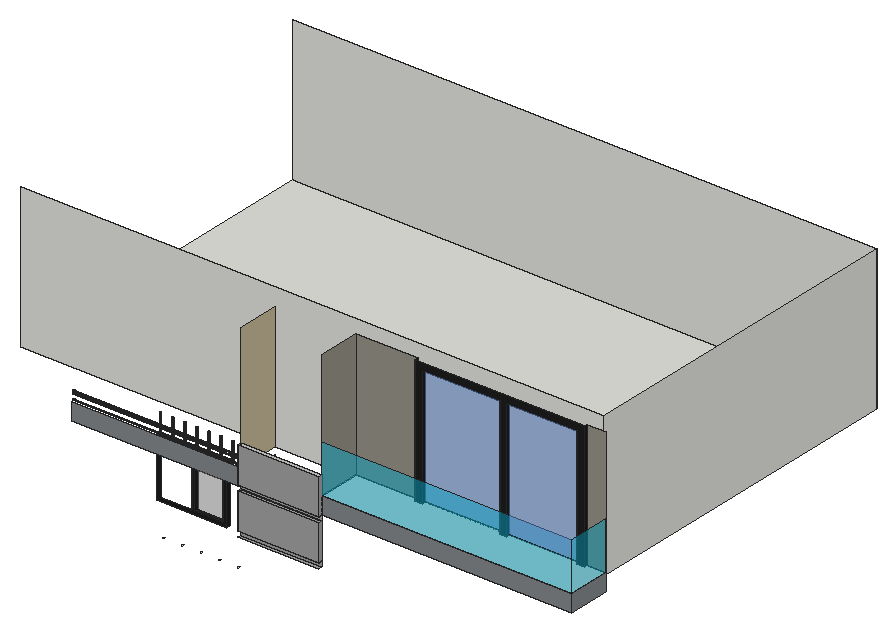
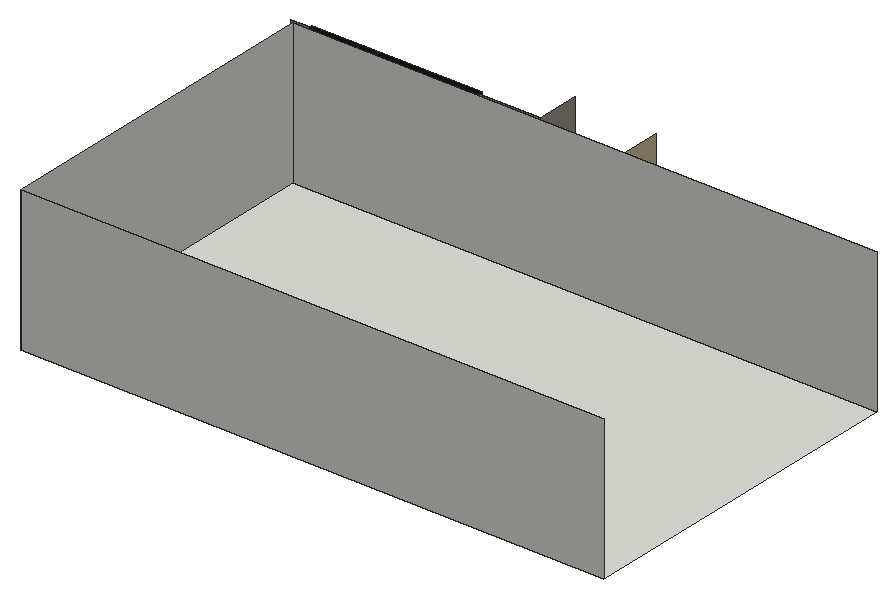
# SketchUp Ruby script. Lengths in inches.
U = 1.inch
M = Sketchup.active_model
def pt(a) = Geom::Point3d.new(a.map { |v| v * U })
def face(e, loops, mat)
  f = e.add_face(loops[0].map { |a| pt(a) })
  loops[1..].each { |l| e.add_face(l.map { |a| pt(a) }).erase! }
  f.material = f.back_material = mat if mat
  f
end
# faces: each face lists its corners as indices into pts; further lists are holes
def faces(e, pts, list, mat = nil) = list.each { |f| face(e, (f[0].is_a?(Array) ? f : [f]).map { |l| l.map { |i| pts[i] } }, mat) }
# xy, xz, yz: faces in a plane at the given z, y or x. An outline is a flat list of corners, or four numbers for a rectangle; further outlines are holes
def ring(l) = l.size == 4 ? [[l[0], l[1]], [l[2], l[1]], [l[2], l[3]], [l[0], l[3]]] : l.each_slice(2).to_a
def flat(e, list, mat, &to3) = list.each { |f| face(e, (f[0].is_a?(Array) ? f : [f]).map { |l| ring(l).map { |u, v| to3.(u, v) } }, mat) }
def xy(e, z, list, mat = nil) = flat(e, list, mat) { |x, y| [x, y, z] }
def xz(e, y, list, mat = nil) = flat(e, list, mat) { |x, z| [x, y, z] }
def yz(e, x, list, mat = nil) = flat(e, list, mat) { |y, z| [x, y, z] }
def lines(e, pts, list) = list.each { |a, b| e.add_line(pt(pts[a]), pt(pts[b])) }
# prism: a flat outline (further loops are holes) pulled along v
def prism(e, loops, v, mat = nil)
  f = face(e, loops, mat); d = Geom::Vector3d.new(v.map { |x| x * U })
  f.pushpull(f.normal.samedirection?(d) ? d.length : -d.length)
end
def box(e, o, s, mat = nil) = prism(e, [[o, [o[0] + s[0], o[1], o[2]], [o[0] + s[0], o[1] + s[1], o[2]], [o[0], o[1] + s[1], o[2]]]], [0, 0, s[2]], mat)
def at(x, y, z, deg = 0) = Geom::Transformation.translation(pt([x, y, z])) * Geom::Transformation.rotation(ORIGIN, Z_AXIS, deg.degrees)
def axes(o, x, y, z) = Geom::Transformation.new([*x, 0, *y, 0, *z, 0, *pt(o).to_a, 1])
def part(name) = M.definitions.add(name)
# library, detail: a bought-in or finely detailed component or shape, given as its bounding box
def library(name, o, s) = part(name).tap { |d| box(d.entities, o, s) }
def detail(e, o, s) = box(e.add_group.entities, o, s)
def put(e, d, t, mat = nil) = e.add_instance(d, t).tap { |i| i.material = mat if mat }
def group(e, t, mat = nil) = e.add_group.tap { |g| g.transformation = t; g.material = mat if mat }.entities
root = M.entities
M.materials.add("[0133_Gray]").color = [128, 128, 128]
M.materials.add("[Blacktop New]").color = [30, 30, 30]
M.materials.add("[Blacktop Old 01]").color = [132, 136, 139]
M.materials.add("[Formica Graystone]").color = [149, 146, 135]
M.materials.add("[Marble Carrara Gold Floor Tile]").color = [225, 223, 217]
M.materials.add("[Pavers Flagstone Gray]").color = [162, 162, 162]
M.materials.add("[Quartz Light Brown]").color = [199, 184, 152]
M.materials.add("[Translucent Glass Blue]").color = [100, 149, 237]
M.materials["[Translucent Glass Blue]"].alpha = 0.5
M.materials.add("[Translucent Glass Gray]").color = [128, 128, 128]
M.materials["[Translucent Glass Gray]"].alpha = 0.5
M.materials.add("[Translucent Glass Tinted]").color = [8, 201, 241]
M.materials["[Translucent Glass Tinted]"].alpha = 0.48
xy(root,170.77,[[164.56,3.4,164.7,3.4,164.82,3.44,164.93,3.52,165.01,3.61,165.07,3.73,165.1,3.86,165.09,3.99,165.05,4.11,164.98,4.22,164.88,4.31,164.76,4.37,164.64,4.39,164.51,4.39,164.38,4.34,164.27,4.27,164.1875,4.18,164.13,4.06,164.1,3.93,164.11,3.8,164.15,3.68,164.22,3.57,164.32,3.48,164.4375,3.42],[180.19,3.4,180.32,3.4,180.44,3.44,180.55,3.52,180.64,3.61,180.7,3.73,180.72,3.86,180.72,3.99,180.68,4.11,180.6,4.22,180.51,4.31,180.39,4.37,180.26,4.39,180.13,4.39,180.01,4.34,179.9,4.27,179.8125,4.18,179.75,4.06,179.73,3.93,179.73,3.8,179.78,3.68,179.85,3.57,179.95,3.48,180.0625,3.42],[195.81,3.4,195.95,3.4,196.07,3.44,196.18,3.52,196.26,3.61,196.32,3.73,196.35,3.86,196.34,3.99,196.3,4.11,196.23,4.22,196.13,4.31,196.01,4.37,195.89,4.39,195.76,4.39,195.63,4.34,195.52,4.27,195.4375,4.18,195.38,4.06,195.35,3.93,195.36,3.8,195.4,3.68,195.47,3.57,195.57,3.48,195.6875,3.42],[211.44,3.4,211.57,3.4,211.69,3.44,211.8,3.52,211.89,3.61,211.95,3.73,211.97,3.86,211.97,3.99,211.93,4.11,211.85,4.22,211.76,4.31,211.64,4.37,211.51,4.39,211.38,4.39,211.26,4.34,211.15,4.27,211.0625,4.18,211,4.06,210.98,3.93,210.98,3.8,211.03,3.68,211.1,3.57,211.2,3.48,211.3125,3.42],[227.06,3.4,227.2,3.4,227.32,3.44,227.43,3.52,227.51,3.61,227.57,3.73,227.6,3.86,227.59,3.99,227.55,4.11,227.48,4.22,227.38,4.31,227.26,4.37,227.14,4.39,227.01,4.39,226.88,4.34,226.77,4.27,226.6875,4.18,226.63,4.06,226.6,3.93,226.61,3.8,226.65,3.68,226.72,3.57,226.82,3.48,226.9375,3.42]])
xy(root,173.78,[[133.06,36,191.5,39]],"[Blacktop New]")
xy(root,176.78,[[164.73,36,188.5,39]],"[Blacktop New]")
xy(root,195.875,[[229.62,0,297.58,3]],"[Pavers Flagstone Gray]")
xy(root,200.56,[[229.62,0,297.58,3]],"[Pavers Flagstone Gray]")
xy(root,220.84,[[164.73,36,188.5,39]],"[Blacktop New]")
xy(root,223.84,[[133.06,36,191.5,39]],"[Blacktop New]")
xy(root,229.1875,[[420.16,36,423.8,39]])
xy(root,229.1875,[[355.33,36,420.16,39],[423.8,36,485,39]],"[Blacktop New]")
xy(root,230.4375,[[229.62,0,297.58,3]],"[Pavers Flagstone Gray]")
xy(root,235.12,[[229.62,0,297.58,3]],"[Pavers Flagstone Gray]")
xy(root,235.1875,[[349.33,36,491,39]])
xy(root,235.1875,[[297.58,3,297.58,39,349.33,39,349.33,36,491,36,491,39,506.625,39,506.625,3]],"[Blacktop Old 01]")
xy(root,240,[[9,48,497.625,333.4375]])
xy(root,246.23,[[231.98,3.83,232.14,3.85,232.29,3.92,232.42,4.02,232.52,4.15,232.58,4.3,232.6,4.46,232.58,4.62,232.52,4.77,232.42,4.9,232.29,5,232.14,5.0625,231.98,5.08,231.82,5.0625,231.67,5,231.54,4.9,231.4375,4.77,231.375,4.62,231.35,4.46,231.375,4.3,231.4375,4.15,231.54,4.02,231.67,3.92,231.82,3.85],[242.1,3.83,242.27,3.85,242.42,3.92,242.55,4.02,242.65,4.15,242.71,4.3,242.73,4.46,242.71,4.62,242.65,4.77,242.55,4.9,242.42,5,242.27,5.0625,242.1,5.08,241.94,5.0625,241.79,5,241.66,4.9,241.5625,4.77,241.5,4.62,241.48,4.46,241.5,4.3,241.5625,4.15,241.66,4.02,241.79,3.92,241.94,3.85],[252.23,3.83,252.39,3.85,252.54,3.92,252.67,4.02,252.77,4.15,252.83,4.3,252.85,4.46,252.83,4.62,252.77,4.77,252.67,4.9,252.54,5,252.39,5.0625,252.23,5.08,252.07,5.0625,251.92,5,251.79,4.9,251.6875,4.77,251.625,4.62,251.6,4.46,251.625,4.3,251.6875,4.15,251.79,4.02,251.92,3.92,252.07,3.85],[262.35,3.83,262.52,3.85,262.67,3.92,262.8,4.02,262.9,4.15,262.96,4.3,262.98,4.46,262.96,4.62,262.9,4.77,262.8,4.9,262.67,5,262.52,5.0625,262.35,5.08,262.19,5.0625,262.04,5,261.91,4.9,261.8125,4.77,261.75,4.62,261.73,4.46,261.75,4.3,261.8125,4.15,261.91,4.02,262.04,3.92,262.19,3.85]])
xy(root,249.45,[[349.33,36,355.33,39],[420.16,36,425.68,39],[485,36,491,39]])
xy(root,249.45,[[297.58,3,506.625,3,506.625,39,491,39,491,36,485,36,485,39,425.68,39,425.68,36,420.16,36,420.16,39,355.33,39,355.33,36,349.33,36,349.33,39,297.58,39]],"[Marble Carrara Gold Floor Tile]")
xz(root,0,[[229.62,200.56,297.58,230.4375],[229.62,235.12,297.58,265]],"[Pavers Flagstone Gray]")
xz(root,3,[[229.62,200.56,297.58,230.4375],[229.62,235.12,297.58,265]])
xz(root,3,[[88.53,232,229.62,246.23],[297.58,235.1875,506.625,249.45]],"[Blacktop Old 01]")
xz(root,3,[[229.62,195.875,297.58,200.56],[229.62,230.4375,297.58,235.12]],"[Pavers Flagstone Gray]")
xz(root,3,[[297.58,249.45,506.625,290.01]],"[Translucent Glass Tinted]")
xz(root,36,[[[133.06,173.78,191.5,223.84],[136.06,176.78,162.28,220.84],[164.73,176.78,188.5,220.84]],[349.33,249.45,355.33,249.45,355.33,349.1875,420.16,349.1875,420.16,249.45,425.68,249.45,425.68,349.1875,485,349.1875,485,249.45,491,249.45,491,355.1875,349.33,355.1875]],"[Blacktop New]")
xz(root,39,[[297.58,235.1875,506.625,239.9375],[297.58,239.9375,506.625,249.45]])
xz(root,39,[[297.58,249.45,349.33,355.1875],[491,249.45,506.625,355.1875]],"[Formica Graystone]")
xz(root,39,[[355.33,249.45,420.16,349.1875],[425.68,249.45,485,349.1875]],"[Translucent Glass Blue]")
xz(root,39,[[164.73,176.78,188.5,220.84]],"[Translucent Glass Gray]")
xz(root,48,[[9,240,497.625,360]])
xz(root,333.4375,[[9,240,497.625,360]])
yz(root,162.28,[[36,176.78,39,220.84]],"[Blacktop New]")
yz(root,164.73,[[36,176.78,39,220.84]],"[Blacktop New]")
yz(root,188.5,[[36,176.78,39,220.84]],"[Blacktop New]")
yz(root,191.5,[[36,173.78,39,223.84]],"[Blacktop New]")
yz(root,229.62,[[3,232,39,240],[3,240,39,240.1875]])
yz(root,229.62,[[0,200.56,3,230.4375],[0,235.12,3,265]],"[Pavers Flagstone Gray]")
yz(root,229.62,[[[3,246.23,39,351.5625],[3.53,262.01,3.625,262.03,3.71,262.0625,3.79,262.12,3.85,262.2,3.89,262.29,3.9,262.39,3.89,262.48,3.85,262.58,3.79,262.65,3.71,262.71,3.625,262.75,3.53,262.76,3.43,262.75,3.34,262.71,3.26,262.65,3.2,262.58,3.16,262.48,3.15,262.39,3.16,262.29,3.2,262.2,3.26,262.12,3.34,262.0625,3.43,262.03],[3.53,260.45,3.625,260.46,3.71,260.5,3.79,260.56,3.85,260.64,3.89,260.73,3.9,260.83,3.89,260.92,3.85,261.01,3.79,261.09,3.71,261.15,3.625,261.1875,3.53,261.2,3.43,261.1875,3.34,261.15,3.26,261.09,3.2,261.01,3.16,260.92,3.15,260.83,3.16,260.73,3.2,260.64,3.26,260.56,3.34,260.5,3.43,260.46],[3.53,258.89,3.625,258.9,3.71,258.9375,3.79,259,3.85,259.08,3.89,259.17,3.9,259.26,3.89,259.36,3.85,259.45,3.79,259.53,3.71,259.59,3.625,259.625,3.53,259.64,3.43,259.625,3.34,259.59,3.26,259.53,3.2,259.45,3.16,259.36,3.15,259.26,3.16,259.17,3.2,259.08,3.26,259,3.34,258.9375,3.43,258.9],[3.53,257.33,3.625,257.34,3.71,257.375,3.79,257.43,3.85,257.51,3.89,257.6,3.9,257.7,3.89,257.8,3.85,257.89,3.79,257.97,3.71,258.02,3.625,258.0625,3.53,258.08,3.43,258.0625,3.34,258.02,3.26,257.97,3.2,257.89,3.16,257.8,3.15,257.7,3.16,257.6,3.2,257.51,3.26,257.43,3.34,257.375,3.43,257.34],[3.53,249.51,3.625,249.53,3.71,249.5625,3.79,249.62,3.85,249.7,3.89,249.79,3.9,249.89,3.89,249.98,3.85,250.08,3.79,250.15,3.71,250.21,3.625,250.25,3.53,250.26,3.43,250.25,3.34,250.21,3.26,250.15,3.2,250.08,3.16,249.98,3.15,249.89,3.16,249.79,3.2,249.7,3.26,249.62,3.34,249.5625,3.43,249.53],[3.53,251.08,3.625,251.09,3.71,251.125,3.79,251.18,3.85,251.26,3.89,251.35,3.9,251.45,3.89,251.55,3.85,251.64,3.79,251.72,3.71,251.77,3.625,251.8125,3.53,251.83,3.43,251.8125,3.34,251.77,3.26,251.72,3.2,251.64,3.16,251.55,3.15,251.45,3.16,251.35,3.2,251.26,3.26,251.18,3.34,251.125,3.43,251.09]]],"[Quartz Light Brown]")
yz(root,229.85,[[3.53,255.76,3.625,255.78,3.71,255.8125,3.79,255.87,3.85,255.95,3.89,256.04,3.9,256.14,3.89,256.23,3.85,256.33,3.79,256.4,3.71,256.46,3.625,256.5,3.53,256.51,3.43,256.5,3.34,256.46,3.26,256.4,3.2,256.33,3.16,256.23,3.15,256.14,3.16,256.04,3.2,255.95,3.26,255.87,3.34,255.8125,3.43,255.78]])
yz(root,231.78,[[3.53,254.2,3.625,254.21,3.71,254.25,3.79,254.31,3.85,254.39,3.89,254.48,3.9,254.58,3.89,254.67,3.85,254.76,3.79,254.84,3.71,254.9,3.625,254.9375,3.53,254.95,3.43,254.9375,3.34,254.9,3.26,254.84,3.2,254.76,3.16,254.67,3.15,254.58,3.16,254.48,3.2,254.39,3.26,254.31,3.34,254.25,3.43,254.21]])
yz(root,231.85,[[3.53,252.64,3.625,252.65,3.71,252.6875,3.79,252.75,3.85,252.83,3.89,252.92,3.9,253.01,3.89,253.11,3.85,253.2,3.79,253.28,3.71,253.34,3.625,253.375,3.53,253.39,3.43,253.375,3.34,253.34,3.26,253.28,3.2,253.2,3.16,253.11,3.15,253.01,3.16,252.92,3.2,252.83,3.26,252.75,3.34,252.6875,3.43,252.65]])
yz(root,232.16,[[3.53,247.95,3.625,247.96,3.71,248,3.79,248.06,3.85,248.14,3.89,248.23,3.9,248.33,3.89,248.42,3.85,248.51,3.79,248.59,3.71,248.65,3.625,248.6875,3.53,248.7,3.43,248.6875,3.34,248.65,3.26,248.59,3.2,248.51,3.16,248.42,3.15,248.33,3.16,248.23,3.2,248.14,3.26,248.06,3.34,248,3.43,247.96]])
yz(root,297.58,[[0,200.56,3,200.625],[0,235.12,3,235.1875],[3,235.1875,39,249.45]])
yz(root,297.58,[[3,249.45,39,355.1875]],"[Formica Graystone]")
yz(root,297.58,[[0,200.625,3,230.4375],[0,235.1875,3,265]],"[Pavers Flagstone Gray]")
yz(root,349.33,[[36,249.45,39,355.1875]],"[Blacktop New]")
yz(root,355.33,[[36,249.45,39,349.1875]],"[Blacktop New]")
yz(root,420.16,[[36,249.45,39,349.1875]],"[Blacktop New]")
yz(root,425.68,[[36,249.45,39,349.1875]],"[Blacktop New]")
yz(root,485,[[36,249.45,39,349.1875]],"[Blacktop New]")
yz(root,491,[[36,249.45,39,355.1875]],"[Blacktop New]")
yz(root,497.625,[[48,240,333.4375,360]])
yz(root,506.625,[[3,235.1875,39,249.45]],"[Blacktop Old 01]")
yz(root,506.625,[[3,249.45,39,290.04]],"[Translucent Glass Tinted]")
p = [[160.94,3.85,246.23],[161.1,3.83,246.23],[161.1,3.83,263.16],[160.94,3.85,263.16],[161.27,3.85,246.23],[161.27,3.85,263.16],
  [171.07,3.85,246.23],[171.23,3.83,246.23],[171.23,3.83,263.16],[171.07,3.85,263.16],[171.39,3.85,246.23],[171.39,3.85,263.16],
  [181.19,3.85,246.23],[181.35,3.83,246.23],[181.35,3.83,263.16],[181.19,3.85,263.16],[181.52,3.85,246.23],[181.52,3.85,263.16],
  [191.32,3.85,246.23],[191.48,3.83,246.23],[191.48,3.83,263.16],[191.32,3.85,263.16],[191.64,3.85,246.23],[191.64,3.85,263.16],
  [201.44,3.85,246.23],[201.6,3.83,246.23],[201.6,3.83,263.16],[201.44,3.85,263.16],[201.77,3.85,246.23],[201.77,3.85,263.16],
  [211.57,3.85,246.23],[211.73,3.83,246.23],[211.73,3.83,263.16],[211.57,3.85,263.16],[211.89,3.85,246.23],[211.89,3.85,263.16],
  [221.69,3.85,246.23],[221.85,3.83,246.23],[221.85,3.83,263.16],[221.69,3.85,263.16],[222.02,3.85,246.23],[222.02,3.85,263.16],
  [160.66,4.02,246.23],[160.79,3.92,246.23],[160.79,3.92,263.16],[160.66,4.02,263.16],[161.42,3.92,246.23],[161.42,3.92,263.16],
  [161.55,4.02,246.23],[161.55,4.02,263.16],[170.79,4.02,246.23],[170.92,3.92,246.23],[170.92,3.92,263.16],[170.79,4.02,263.16],
  [171.54,3.92,246.23],[171.54,3.92,263.16],[171.67,4.02,246.23],[171.67,4.02,263.16],[180.91,4.02,246.23],[181.04,3.92,246.23],
  [181.04,3.92,263.16],[180.91,4.02,263.16],[181.67,3.92,246.23],[181.67,3.92,263.16],[181.8,4.02,246.23],[181.8,4.02,263.16],
  [191.04,4.02,246.23],[191.17,3.92,246.23],[191.17,3.92,263.16],[191.04,4.02,263.16],[191.79,3.92,246.23],[191.79,3.92,263.16],
  [191.92,4.02,246.23],[191.92,4.02,263.16],[201.16,4.02,246.23],[201.29,3.92,246.23],[201.29,3.92,263.16],[201.16,4.02,263.16],
  [201.92,3.92,246.23],[201.92,3.92,263.16],[202.05,4.02,246.23],[202.05,4.02,263.16],[211.29,4.02,246.23],[211.42,3.92,246.23],
  [211.42,3.92,263.16],[211.29,4.02,263.16],[212.04,3.92,246.23],[212.04,3.92,263.16],[212.17,4.02,246.23],[212.17,4.02,263.16],
  [221.41,4.02,246.23],[221.54,3.92,246.23],[221.54,3.92,263.16],[221.41,4.02,263.16],[222.17,3.92,246.23],[222.17,3.92,263.16],
  [222.3,4.02,246.23],[222.3,4.02,263.16],[160.5625,4.15,246.23],[160.5625,4.15,263.16],[161.65,4.15,246.23],[161.65,4.15,263.16],
  [170.6875,4.15,246.23],[170.6875,4.15,263.16],[171.77,4.15,246.23],[171.77,4.15,263.16],[180.8125,4.15,246.23],[180.8125,4.15,263.16],
  [181.9,4.15,246.23],[181.9,4.15,263.16],[190.9375,4.15,246.23],[190.9375,4.15,263.16],[192.02,4.15,246.23],[192.02,4.15,263.16],
  [201.0625,4.15,246.23],[201.0625,4.15,263.16],[202.15,4.15,246.23],[202.15,4.15,263.16],[211.1875,4.15,246.23],[211.1875,4.15,263.16],
  [212.27,4.15,246.23],[212.27,4.15,263.16],[221.3125,4.15,246.23],[221.3125,4.15,263.16],[222.4,4.15,246.23],[222.4,4.15,263.16],
  [160.5,4.3,246.23],[160.5,4.3,263.16],[161.71,4.3,246.23],[161.71,4.3,263.16],[170.625,4.3,246.23],[170.625,4.3,263.16],
  [171.83,4.3,246.23],[171.83,4.3,263.16],[180.75,4.3,246.23],[180.75,4.3,263.16],[181.96,4.3,246.23],[181.96,4.3,263.16],
  [190.875,4.3,246.23],[190.875,4.3,263.16],[192.08,4.3,246.23],[192.08,4.3,263.16],[201,4.3,246.23],[201,4.3,263.16],
  [202.21,4.3,246.23],[202.21,4.3,263.16],[211.125,4.3,246.23],[211.125,4.3,263.16],[212.33,4.3,246.23],[212.33,4.3,263.16],
  [221.25,4.3,246.23],[221.25,4.3,263.16],[222.46,4.3,246.23],[222.46,4.3,263.16],[160.48,4.46,246.23],[160.48,4.46,263.16],
  [161.73,4.46,246.23],[161.73,4.46,263.16],[170.6,4.46,246.23],[170.6,4.46,263.16],[171.85,4.46,246.23],[171.85,4.46,263.16],
  [180.73,4.46,246.23],[180.73,4.46,263.16],[181.98,4.46,246.23],[181.98,4.46,263.16],[190.85,4.46,246.23],[190.85,4.46,263.16],
  [192.1,4.46,246.23],[192.1,4.46,263.16],[200.98,4.46,246.23],[200.98,4.46,263.16],[202.23,4.46,246.23],[202.23,4.46,263.16],
  [211.1,4.46,246.23],[211.1,4.46,263.16],[212.35,4.46,246.23],[212.35,4.46,263.16],[221.23,4.46,246.23],[221.23,4.46,263.16],
  [222.48,4.46,246.23],[222.48,4.46,263.16],[160.5,4.62,246.23],[160.5,4.62,263.16],[161.71,4.62,246.23],[161.71,4.62,263.16],
  [170.625,4.62,246.23],[170.625,4.62,263.16],[171.83,4.62,246.23],[171.83,4.62,263.16],[180.75,4.62,246.23],[180.75,4.62,263.16],
  [181.96,4.62,246.23],[181.96,4.62,263.16],[190.875,4.62,246.23],[190.875,4.62,263.16],[192.08,4.62,246.23],[192.08,4.62,263.16],
  [201,4.62,246.23],[201,4.62,263.16],[202.21,4.62,246.23],[202.21,4.62,263.16],[211.125,4.62,246.23],[211.125,4.62,263.16],
  [212.33,4.62,246.23],[212.33,4.62,263.16],[221.25,4.62,246.23],[221.25,4.62,263.16],[222.46,4.62,246.23],[222.46,4.62,263.16],
  [160.5625,4.77,246.23],[160.5625,4.77,263.16],[161.65,4.77,246.23],[161.65,4.77,263.16],[170.6875,4.77,246.23],[170.6875,4.77,263.16],
  [171.77,4.77,246.23],[171.77,4.77,263.16],[180.8125,4.77,246.23],[180.8125,4.77,263.16],[181.9,4.77,246.23],[181.9,4.77,263.16],
  [190.9375,4.77,246.23],[190.9375,4.77,263.16],[192.02,4.77,246.23],[192.02,4.77,263.16],[201.0625,4.77,246.23],[201.0625,4.77,263.16],
  [202.15,4.77,246.23],[202.15,4.77,263.16],[211.1875,4.77,246.23],[211.1875,4.77,263.16],[212.27,4.77,246.23],[212.27,4.77,263.16],
  [221.3125,4.77,246.23],[221.3125,4.77,263.16],[222.4,4.77,246.23],[222.4,4.77,263.16],[160.66,4.9,246.23],[160.66,4.9,263.16],
  [161.55,4.9,246.23],[161.55,4.9,263.16],[170.79,4.9,246.23],[170.79,4.9,263.16],[171.67,4.9,246.23],[171.67,4.9,263.16],
  [180.91,4.9,246.23],[180.91,4.9,263.16],[181.8,4.9,246.23],[181.8,4.9,263.16],[191.04,4.9,246.23],[191.04,4.9,263.16],
  [191.92,4.9,246.23],[191.92,4.9,263.16],[201.16,4.9,246.23],[201.16,4.9,263.16],[202.05,4.9,246.23],[202.05,4.9,263.16],
  [211.29,4.9,246.23],[211.29,4.9,263.16],[212.17,4.9,246.23],[212.17,4.9,263.16],[221.41,4.9,246.23],[221.41,4.9,263.16],
  [222.3,4.9,246.23],[222.3,4.9,263.16],[160.79,5,246.23],[160.79,5,263.16],[161.42,5,246.23],[161.42,5,263.16],
  [170.92,5,246.23],[170.92,5,263.16],[171.54,5,246.23],[171.54,5,263.16],[181.04,5,246.23],[181.04,5,263.16],
  [181.67,5,246.23],[181.67,5,263.16],[191.17,5,246.23],[191.17,5,263.16],[191.79,5,246.23],[191.79,5,263.16],
  [201.29,5,246.23],[201.29,5,263.16],[201.92,5,246.23],[201.92,5,263.16],[211.42,5,246.23],[211.42,5,263.16],
  [212.04,5,246.23],[212.04,5,263.16],[221.54,5,246.23],[221.54,5,263.16],[222.17,5,246.23],[222.17,5,263.16],
  [160.94,5.0625,246.23],[160.94,5.0625,263.16],[161.27,5.0625,246.23],[161.27,5.0625,263.16],[171.07,5.0625,246.23],[171.07,5.0625,263.16],
  [171.39,5.0625,246.23],[171.39,5.0625,263.16],[181.19,5.0625,246.23],[181.19,5.0625,263.16],[181.52,5.0625,246.23],[181.52,5.0625,263.16],
  [191.32,5.0625,246.23],[191.32,5.0625,263.16],[191.64,5.0625,246.23],[191.64,5.0625,263.16],[201.44,5.0625,246.23],[201.44,5.0625,263.16],
  [201.77,5.0625,246.23],[201.77,5.0625,263.16],[211.57,5.0625,246.23],[211.57,5.0625,263.16],[211.89,5.0625,246.23],[211.89,5.0625,263.16],
  [221.69,5.0625,246.23],[221.69,5.0625,263.16],[222.02,5.0625,246.23],[222.02,5.0625,263.16],[161.1,5.08,246.23],[161.1,5.08,263.16],
  [171.23,5.08,246.23],[171.23,5.08,263.16],[181.35,5.08,246.23],[181.35,5.08,263.16],[191.48,5.08,246.23],[191.48,5.08,263.16],
  [201.6,5.08,246.23],[201.6,5.08,263.16],[211.73,5.08,246.23],[211.73,5.08,263.16],[221.85,5.08,246.23],[221.85,5.08,263.16],
  [88.53,3.34,248],[88.53,3.43,247.96],[232.16,3.43,247.96],[232.16,3.34,248],[88.53,3.26,248.06],[232.16,3.26,248.06],
  [88.53,3.53,247.95],[232.16,3.53,247.95],[88.53,3.625,247.96],[232.16,3.625,247.96],[88.53,3.71,248],[232.16,3.71,248],
  [88.53,3.79,248.06],[232.16,3.79,248.06],[88.53,3.2,248.14],[232.16,3.2,248.14],[88.53,3.16,248.23],[232.16,3.16,248.23],
  [88.53,3.85,248.14],[232.16,3.85,248.14],[88.53,3.89,248.23],[232.16,3.89,248.23],[88.53,3.15,248.33],[232.16,3.15,248.33],
  [88.53,3.9,248.33],[232.16,3.9,248.33],[88.53,3.16,248.42],[232.16,3.16,248.42],[88.53,3.89,248.42],[232.16,3.89,248.42],
  [88.53,3.2,248.51],[232.16,3.2,248.51],[88.53,3.85,248.51],[232.16,3.85,248.51],[88.53,3.26,248.59],[232.16,3.26,248.59],
  [88.53,3.79,248.59],[232.16,3.79,248.59],[88.53,3.34,248.65],[232.16,3.34,248.65],[88.53,3.43,248.6875],[232.16,3.43,248.6875],
  [88.53,3.71,248.65],[88.53,3.625,248.6875],[232.16,3.625,248.6875],[232.16,3.71,248.65],[88.53,3.53,248.7],[232.16,3.53,248.7],
  [88.53,3.43,252.65],[88.53,3.53,252.64],[231.85,3.53,252.64],[231.85,3.43,252.65],[88.53,3.625,252.65],[231.85,3.625,252.65],
  [88.53,3.2,252.83],[88.53,3.26,252.75],[231.85,3.26,252.75],[231.85,3.2,252.83],[88.53,3.34,252.6875],[231.85,3.34,252.6875],
  [88.53,3.71,252.6875],[231.85,3.71,252.6875],[88.53,3.79,252.75],[231.85,3.79,252.75],[88.53,3.85,252.83],[231.85,3.85,252.83],
  [88.53,3.16,252.92],[231.85,3.16,252.92],[88.53,3.89,252.92],[231.85,3.89,252.92],[88.53,3.15,253.01],[231.85,3.15,253.01],
  [88.53,3.9,253.01],[231.85,3.9,253.01],[88.53,3.16,253.11],[231.85,3.16,253.11],[88.53,3.89,253.11],[231.85,3.89,253.11],
  [88.53,3.2,253.2],[231.85,3.2,253.2],[88.53,3.85,253.2],[231.85,3.85,253.2],[88.53,3.26,253.28],[231.85,3.26,253.28],
  [88.53,3.79,253.28],[231.85,3.79,253.28],[88.53,3.34,253.34],[231.85,3.34,253.34],[88.53,3.43,253.375],[231.85,3.43,253.375],
  [88.53,3.71,253.34],[88.53,3.625,253.375],[231.85,3.625,253.375],[231.85,3.71,253.34],[88.53,3.53,253.39],[231.85,3.53,253.39],
  [88.53,3.26,254.84],[88.53,3.2,254.76],[231.78,3.2,254.76],[231.78,3.26,254.84],[88.53,3.34,254.9],[231.78,3.34,254.9],
  [88.53,3.79,254.84],[88.53,3.71,254.9],[231.78,3.71,254.9],[231.78,3.79,254.84],[88.53,3.85,254.76],[231.78,3.85,254.76],
  [88.53,3.43,254.9375],[231.78,3.43,254.9375],[88.53,3.53,254.95],[231.78,3.53,254.95],[88.53,3.625,254.9375],[231.78,3.625,254.9375]]
faces(root,p,[[0,1,2,3],[1,4,5,2],[6,7,8,9],[7,10,11,8],[12,13,14,15],[13,16,17,14],[18,19,20,21],[19,22,23,20],
  [24,25,26,27],[25,28,29,26],[30,31,32,33],[31,34,35,32],[36,37,38,39],[37,40,41,38],[42,43,44,45],[43,0,3,44],
  [4,46,47,5],[46,48,49,47],[50,51,52,53],[51,6,9,52],[10,54,55,11],[54,56,57,55],[58,59,60,61],[59,12,15,60],
  [16,62,63,17],[62,64,65,63],[66,67,68,69],[67,18,21,68],[22,70,71,23],[70,72,73,71],[74,75,76,77],[75,24,27,76],
  [28,78,79,29],[78,80,81,79],[82,83,84,85],[83,30,33,84],[34,86,87,35],[86,88,89,87],[90,91,92,93],[91,36,39,92],
  [40,94,95,41],[94,96,97,95],[98,42,45,99],[48,100,101,49],[102,50,53,103],[56,104,105,57],[106,58,61,107],[64,108,109,65],
  [110,66,69,111],[72,112,113,73],[114,74,77,115],[80,116,117,81],[118,82,85,119],[88,120,121,89],[122,90,93,123],[96,124,125,97],
  [126,98,99,127],[100,128,129,101],[130,102,103,131],[104,132,133,105],[134,106,107,135],[108,136,137,109],[138,110,111,139],[112,140,141,113],
  [142,114,115,143],[116,144,145,117],[146,118,119,147],[120,148,149,121],[150,122,123,151],[124,152,153,125],[154,126,127,155],[128,156,157,129],
  [158,130,131,159],[132,160,161,133],[162,134,135,163],[136,164,165,137],[166,138,139,167],[140,168,169,141],[170,142,143,171],[144,172,173,145],
  [174,146,147,175],[148,176,177,149],[178,150,151,179],[152,180,181,153],[182,154,155,183],[156,184,185,157],[186,158,159,187],[160,188,189,161],
  [190,162,163,191],[164,192,193,165],[194,166,167,195],[168,196,197,169],[198,170,171,199],[172,200,201,173],[202,174,175,203],[176,204,205,177],
  [206,178,179,207],[180,208,209,181],[210,182,183,211],[184,212,213,185],[214,186,187,215],[188,216,217,189],[218,190,191,219],[192,220,221,193],
  [222,194,195,223],[196,224,225,197],[226,198,199,227],[200,228,229,201],[230,202,203,231],[204,232,233,205],[234,206,207,235],[208,236,237,209],
  [238,210,211,239],[212,240,241,213],[242,214,215,243],[216,244,245,217],[246,218,219,247],[220,248,249,221],[250,222,223,251],[224,252,253,225],
  [254,226,227,255],[228,256,257,229],[258,230,231,259],[232,260,261,233],[262,234,235,263],[236,264,265,237],[266,238,239,267],[240,268,269,241],
  [270,242,243,271],[244,272,273,245],[274,246,247,275],[248,276,277,249],[278,250,251,279],[252,280,281,253],[282,254,255,283],[256,284,285,257],
  [286,258,259,287],[260,288,289,261],[290,262,263,291],[264,292,293,265],[294,266,267,295],[268,296,297,269],[298,270,271,299],[272,300,301,273],
  [302,274,275,303],[276,304,305,277],[306,278,279,307],[280,308,309,281],[310,282,283,311],[284,312,313,285],[314,286,287,315],[288,316,317,289],
  [318,290,291,319],[292,320,321,293],[322,294,295,323],[296,322,323,297],[324,298,299,325],[300,324,325,301],[326,302,303,327],[304,326,327,305],
  [328,306,307,329],[308,328,329,309],[330,310,311,331],[312,330,331,313],[332,314,315,333],[316,332,333,317],[334,318,319,335],[320,334,335,321],
  [336,337,338,339],[340,336,339,341],[337,342,343,338],[342,344,345,343],[344,346,347,345],[346,348,349,347],[350,340,341,351],[352,350,351,353],
  [348,354,355,349],[354,356,357,355],[358,352,353,359],[356,360,361,357],[362,358,359,363],[360,364,365,361],[366,362,363,367],[364,368,369,365],
  [370,366,367,371],[368,372,373,369],[374,370,371,375],[376,374,375,377],[378,379,380,381],[372,378,381,373],[382,376,377,383],[379,382,383,380],
  [384,385,386,387],[385,388,389,386],[390,391,392,393],[394,384,387,395],[391,394,395,392],[388,396,397,389],[396,398,399,397],[398,400,401,399],
  [402,390,393,403],[400,404,405,401],[406,402,403,407],[404,408,409,405],[410,406,407,411],[408,412,413,409],[414,410,411,415],[412,416,417,413],
  [418,414,415,419],[416,420,421,417],[422,418,419,423],[424,422,423,425],[426,427,428,429],[420,426,429,421],[430,424,425,431],[427,430,431,428],
  [432,433,434,435],[436,432,435,437],[438,439,440,441],[442,438,441,443],[444,436,437,445],[446,444,445,447],[448,446,447,449],[439,448,449,440]],"[0133_Gray]")
